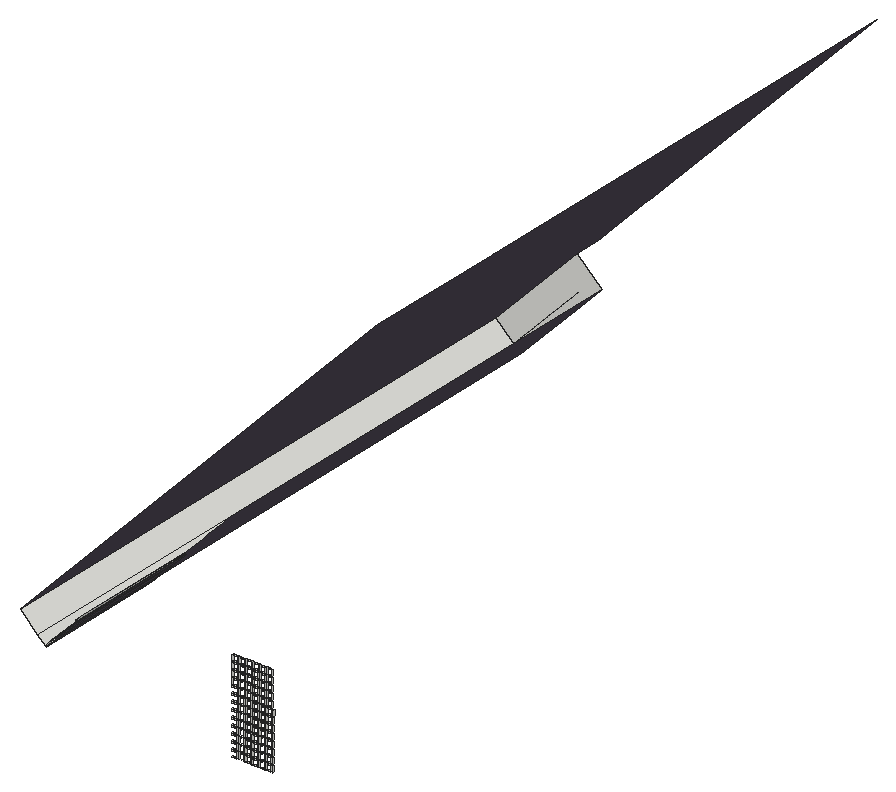
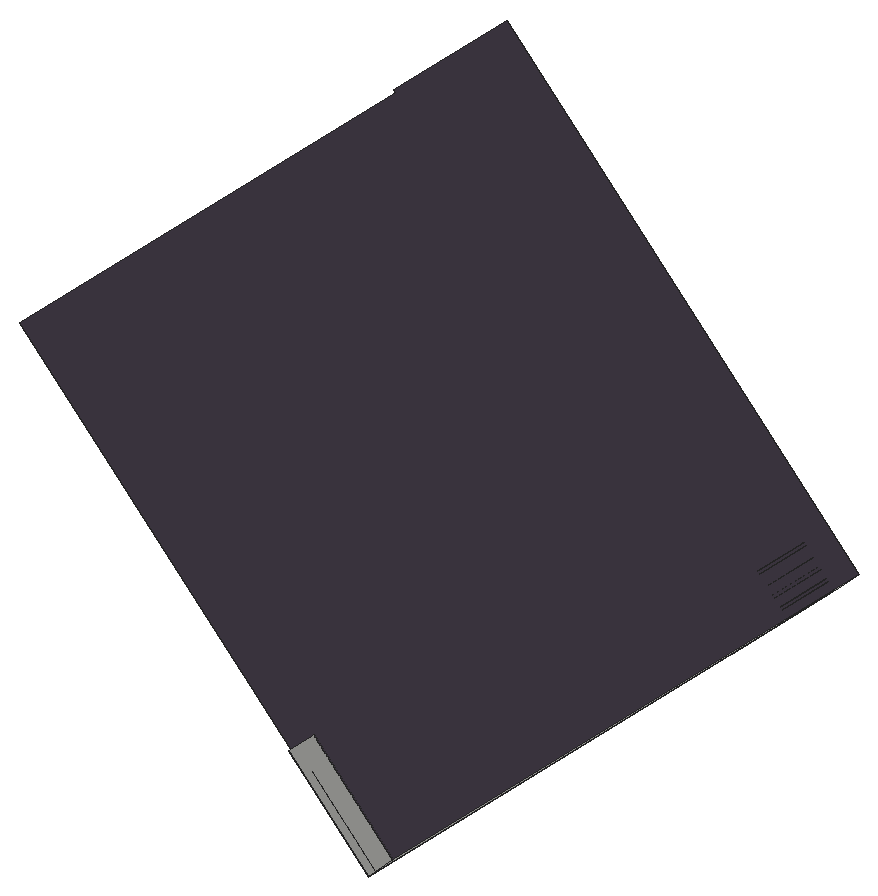
# SketchUp Ruby script. Lengths in inches.
U = 1.inch
M = Sketchup.active_model
def pt(a) = Geom::Point3d.new(a.map { |v| v * U })
def face(e, loops, mat)
  f = e.add_face(loops[0].map { |a| pt(a) })
  loops[1..].each { |l| e.add_face(l.map { |a| pt(a) }).erase! }
  f.material = f.back_material = mat if mat
  f
end
# faces: each face lists its corners as indices into pts; further lists are holes
def faces(e, pts, list, mat = nil) = list.each { |f| face(e, (f[0].is_a?(Array) ? f : [f]).map { |l| l.map { |i| pts[i] } }, mat) }
# xy, xz, yz: faces in a plane at the given z, y or x. An outline is a flat list of corners, or four numbers for a rectangle; further outlines are holes
def ring(l) = l.size == 4 ? [[l[0], l[1]], [l[2], l[1]], [l[2], l[3]], [l[0], l[3]]] : l.each_slice(2).to_a
def flat(e, list, mat, &to3) = list.each { |f| face(e, (f[0].is_a?(Array) ? f : [f]).map { |l| ring(l).map { |u, v| to3.(u, v) } }, mat) }
def xy(e, z, list, mat = nil) = flat(e, list, mat) { |x, y| [x, y, z] }
def xz(e, y, list, mat = nil) = flat(e, list, mat) { |x, z| [x, y, z] }
def yz(e, x, list, mat = nil) = flat(e, list, mat) { |y, z| [x, y, z] }
def lines(e, pts, list) = list.each { |a, b| e.add_line(pt(pts[a]), pt(pts[b])) }
# prism: a flat outline (further loops are holes) pulled along v
def prism(e, loops, v, mat = nil)
  f = face(e, loops, mat); d = Geom::Vector3d.new(v.map { |x| x * U })
  f.pushpull(f.normal.samedirection?(d) ? d.length : -d.length)
end
def box(e, o, s, mat = nil) = prism(e, [[o, [o[0] + s[0], o[1], o[2]], [o[0] + s[0], o[1] + s[1], o[2]], [o[0], o[1] + s[1], o[2]]]], [0, 0, s[2]], mat)
def at(x, y, z, deg = 0) = Geom::Transformation.translation(pt([x, y, z])) * Geom::Transformation.rotation(ORIGIN, Z_AXIS, deg.degrees)
def axes(o, x, y, z) = Geom::Transformation.new([*x, 0, *y, 0, *z, 0, *pt(o).to_a, 1])
def part(name) = M.definitions.add(name)
# library, detail: a bought-in or finely detailed component or shape, given as its bounding box
def library(name, o, s) = part(name).tap { |d| box(d.entities, o, s) }
def detail(e, o, s) = box(e.add_group.entities, o, s)
def put(e, d, t, mat = nil) = e.add_instance(d, t).tap { |i| i.material = mat if mat }
def group(e, t, mat = nil) = e.add_group.tap { |g| g.transformation = t; g.material = mat if mat }.entities
root = M.entities
M.materials.add("[Color M06]").color = [79, 71, 84]
xy(root,265.77,[[989.38,2332.13,991.69,2332.76],[992.29,2332.13,994.6,2332.76],[995.2,2332.13,997.52,2332.76],[998.12,2332.13,1000.43,2332.76],[1001.03,2332.13,1003.34,2332.76],
  [1003.94,2332.13,1006.25,2332.76]])
xy(root,268.09,[[989.38,2332.13,991.69,2332.76],[992.29,2332.13,994.6,2332.76],[995.2,2332.13,997.52,2332.76],[998.12,2332.13,1000.43,2332.76],[1001.03,2332.13,1003.34,2332.76],
  [1003.94,2332.13,1006.25,2332.76]])
xy(root,268.82,[[989.41,2332.13,991.72,2332.76],[992.32,2332.13,994.63,2332.76],[995.23,2332.13,997.55,2332.76],[998.15,2332.13,1000.46,2332.76],[1001.06,2332.13,1003.37,2332.76],
  [1003.97,2332.13,1006.28,2332.76]])
xy(root,271.13,[[989.41,2332.13,991.72,2332.76],[992.32,2332.13,994.63,2332.76],[995.23,2332.13,997.55,2332.76],[998.15,2332.13,1000.46,2332.76],[1001.06,2332.13,1003.37,2332.76],
  [1003.97,2332.13,1006.28,2332.76]])
xy(root,271.86,[[989.4375,2332.13,991.75,2332.76],[992.35,2332.13,994.66,2332.76],[995.26,2332.13,997.57,2332.76],[998.17,2332.13,1000.49,2332.76],[1001.09,2332.13,1003.4,2332.76],
  [1004,2332.13,1006.3125,2332.76]])
xy(root,274.17,[[989.4375,2332.13,991.75,2332.76],[992.35,2332.13,994.66,2332.76],[995.26,2332.13,997.57,2332.76],[998.17,2332.13,1000.49,2332.76],[1001.09,2332.13,1003.4,2332.76],
  [1004,2332.13,1006.3125,2332.76]])
xy(root,274.91,[[989.47,2332.13,991.78,2332.76],[992.38,2332.13,994.69,2332.76],[995.29,2332.13,997.6,2332.76],[998.2,2332.13,1000.52,2332.76],[1001.12,2332.13,1003.43,2332.76],
  [1004.03,2332.13,1006.34,2332.76]])
xy(root,277.22,[[989.47,2332.13,991.78,2332.76],[992.38,2332.13,994.69,2332.76],[995.29,2332.13,997.6,2332.76],[998.2,2332.13,1000.52,2332.76],[1001.12,2332.13,1003.43,2332.76],
  [1004.03,2332.13,1006.34,2332.76]])
xy(root,277.95,[[989.5,2332.13,991.81,2332.76],[992.41,2332.13,994.72,2332.76],[995.32,2332.13,997.63,2332.76],[998.23,2332.13,1000.55,2332.76],[1001.14,2332.13,1003.46,2332.76],
  [1004.06,2332.13,1006.37,2332.76]])
xy(root,280.26,[[989.5,2332.13,991.81,2332.76],[992.41,2332.13,994.72,2332.76],[995.32,2332.13,997.63,2332.76],[998.23,2332.13,1000.55,2332.76],[1001.14,2332.13,1003.46,2332.76],
  [1004.06,2332.13,1006.37,2332.76]])
xy(root,281,[[989.53,2332.13,991.84,2332.76],[992.4375,2332.13,994.75,2332.76],[995.35,2332.13,997.66,2332.76],[998.26,2332.13,1000.57,2332.76],[1001.17,2332.13,1003.49,2332.76],
  [1004.09,2332.13,1006.4,2332.76]])
xy(root,283.31,[[989.53,2332.13,991.84,2332.76],[992.4375,2332.13,994.75,2332.76],[995.35,2332.13,997.66,2332.76],[998.26,2332.13,1000.57,2332.76],[1001.17,2332.13,1003.49,2332.76],
  [1004.09,2332.13,1006.4,2332.76]])
xy(root,284.04,[[989.55,2332.13,991.87,2332.76],[992.47,2332.13,994.78,2332.76],[995.38,2332.13,997.69,2332.76],[998.29,2332.13,1000.6,2332.76],[1001.2,2332.13,1003.52,2332.76],
  [1004.11,2332.13,1006.43,2332.76]])
xy(root,286.35,[[989.55,2332.13,991.87,2332.76],[992.47,2332.13,994.78,2332.76],[995.38,2332.13,997.69,2332.76],[998.29,2332.13,1000.6,2332.76],[1001.2,2332.13,1003.52,2332.76],
  [1004.11,2332.13,1006.43,2332.76]])
xy(root,287.09,[[989.58,2332.13,991.9,2332.76],[992.5,2332.13,994.81,2332.76],[995.41,2332.13,997.72,2332.76],[998.32,2332.13,1000.63,2332.76],[1001.23,2332.13,1003.54,2332.76],
  [1004.14,2332.13,1006.46,2332.76]])
xy(root,289.4,[[989.58,2332.13,991.9,2332.76],[992.5,2332.13,994.81,2332.76],[995.41,2332.13,997.72,2332.76],[998.32,2332.13,1000.63,2332.76],[1001.23,2332.13,1003.54,2332.76],
  [1004.14,2332.13,1006.46,2332.76]])
xy(root,290.13,[[989.61,2332.13,991.92,2332.76],[992.52,2332.13,994.84,2332.76],[995.4375,2332.13,997.75,2332.76],[998.35,2332.13,1000.66,2332.76],[1001.26,2332.13,1003.57,2332.76],
  [1004.17,2332.13,1006.49,2332.76]])
xy(root,292.44,[[989.61,2332.13,991.92,2332.76],[992.52,2332.13,994.84,2332.76],[995.4375,2332.13,997.75,2332.76],[998.35,2332.13,1000.66,2332.76],[1001.26,2332.13,1003.57,2332.76],
  [1004.17,2332.13,1006.49,2332.76]])
xy(root,293.18,[[989.64,2332.13,991.95,2332.76],[992.55,2332.13,994.87,2332.76],[995.47,2332.13,997.78,2332.76],[998.38,2332.13,1000.69,2332.76],[1001.29,2332.13,1003.6,2332.76],
  [1004.2,2332.13,1006.51,2332.76]])
xy(root,295.49,[[989.64,2332.13,991.95,2332.76],[992.55,2332.13,994.87,2332.76],[995.47,2332.13,997.78,2332.76],[998.38,2332.13,1000.69,2332.76],[1001.29,2332.13,1003.6,2332.76],
  [1004.2,2332.13,1006.51,2332.76]])
xy(root,296.22,[[989.67,2332.13,991.98,2332.76],[992.58,2332.13,994.89,2332.76],[995.49,2332.13,997.81,2332.76],[998.41,2332.13,1000.72,2332.76],[1001.32,2332.13,1003.63,2332.76],
  [1004.23,2332.13,1006.54,2332.76]])
xy(root,298.53,[[989.67,2332.13,991.98,2332.76],[992.58,2332.13,994.89,2332.76],[995.49,2332.13,997.81,2332.76],[998.41,2332.13,1000.72,2332.76],[1001.32,2332.13,1003.63,2332.76],
  [1004.23,2332.13,1006.54,2332.76]])
xy(root,299.27,[[989.7,2332.13,992.01,2332.76],[992.61,2332.13,994.92,2332.76],[995.52,2332.13,997.84,2332.76],[998.44,2332.13,1000.75,2332.76],[1001.35,2332.13,1003.66,2332.76],
  [1004.26,2332.13,1006.57,2332.76]])
xy(root,301.58,[[989.7,2332.13,992.01,2332.76],[992.61,2332.13,994.92,2332.76],[995.52,2332.13,997.84,2332.76],[998.44,2332.13,1000.75,2332.76],[1001.35,2332.13,1003.66,2332.76],
  [1004.26,2332.13,1006.57,2332.76]])
xy(root,302.31,[[989.73,2332.13,992.04,2332.76],[992.64,2332.13,994.95,2332.76],[995.55,2332.13,997.86,2332.76],[998.46,2332.13,1000.78,2332.76],[1001.375,2332.13,1003.6875,2332.76],
  [1004.29,2332.13,1006.6,2332.76]])
xy(root,304.62,[[989.73,2332.13,992.04,2332.76],[992.64,2332.13,994.95,2332.76],[995.55,2332.13,997.86,2332.76],[998.46,2332.13,1000.78,2332.76],[1001.375,2332.13,1003.6875,2332.76],
  [1004.29,2332.13,1006.6,2332.76]])
xz(root,2373.56,[[921.31,289.13,920.85,289.56,923.27,292.13,923.73,291.7],[924.61,292.64,924.15,293.0625,926.57,295.64,927.03,295.21],[927.91,296.14,927.45,296.57,929.87,299.14,930.33,298.71],[931.2,299.64,930.75,300.07,933.17,302.64,933.625,302.22],[934.5,303.15,934.05,303.58,936.47,306.15,936.92,305.72],
  [934.05,303.58,933.82,303.79,936.24,306.36,936.47,306.15]])
xz(root,2571.2,[[920.85,289.56,917.71,292.52,910.18,299.61,944.56,336.13,955.23,326.08,948.3125,318.73]])
yz(root,989.64,[[2332.13,293.18,2332.76,295.49]])
yz(root,989.67,[[2332.13,296.22,2332.76,298.53]])
yz(root,989.7,[[2332.13,299.27,2332.76,301.58]])
yz(root,989.73,[[2332.13,302.31,2332.76,304.62]])
yz(root,991.69,[[2332.13,265.77,2332.76,268.09]])
yz(root,991.72,[[2332.13,268.82,2332.76,271.13]])
yz(root,991.75,[[2332.13,271.86,2332.76,274.17]])
yz(root,991.78,[[2332.13,274.91,2332.76,277.22]])
yz(root,991.81,[[2332.13,277.95,2332.76,280.26]])
yz(root,991.84,[[2332.13,281,2332.76,283.31]])
yz(root,991.87,[[2332.13,284.04,2332.76,286.35]])
yz(root,991.9,[[2332.13,287.09,2332.76,289.4]])
yz(root,991.92,[[2332.13,290.13,2332.76,292.44]])
yz(root,991.95,[[2332.13,293.18,2332.76,295.49]])
yz(root,991.98,[[2332.13,296.22,2332.76,298.53]])
yz(root,992.01,[[2332.13,299.27,2332.76,301.58]])
yz(root,992.04,[[2332.13,302.31,2332.76,304.62]])
yz(root,992.29,[[2332.13,265.77,2332.76,268.09]])
yz(root,992.32,[[2332.13,268.82,2332.76,271.13]])
yz(root,992.35,[[2332.13,271.86,2332.76,274.17]])
yz(root,992.38,[[2332.13,274.91,2332.76,277.22]])
yz(root,992.41,[[2332.13,277.95,2332.76,280.26]])
yz(root,992.4375,[[2332.13,281,2332.76,283.31]])
yz(root,992.47,[[2332.13,284.04,2332.76,286.35]])
yz(root,992.5,[[2332.13,287.09,2332.76,289.4]])
yz(root,992.52,[[2332.13,290.13,2332.76,292.44]])
yz(root,992.55,[[2332.13,293.18,2332.76,295.49]])
yz(root,992.58,[[2332.13,296.22,2332.76,298.53]])
yz(root,992.61,[[2332.13,299.27,2332.76,301.58]])
yz(root,992.64,[[2332.13,302.31,2332.76,304.62]])
yz(root,994.6,[[2332.13,265.77,2332.76,268.09]])
yz(root,994.63,[[2332.13,268.82,2332.76,271.13]])
yz(root,994.66,[[2332.13,271.86,2332.76,274.17]])
yz(root,994.69,[[2332.13,274.91,2332.76,277.22]])
yz(root,994.72,[[2332.13,277.95,2332.76,280.26]])
yz(root,994.75,[[2332.13,281,2332.76,283.31]])
yz(root,994.78,[[2332.13,284.04,2332.76,286.35]])
yz(root,994.81,[[2332.13,287.09,2332.76,289.4]])
yz(root,994.84,[[2332.13,290.13,2332.76,292.44]])
yz(root,994.87,[[2332.13,293.18,2332.76,295.49]])
yz(root,994.89,[[2332.13,296.22,2332.76,298.53]])
yz(root,994.92,[[2332.13,299.27,2332.76,301.58]])
yz(root,994.95,[[2332.13,302.31,2332.76,304.62]])
yz(root,995.2,[[2332.13,265.77,2332.76,268.09]])
yz(root,995.23,[[2332.13,268.82,2332.76,271.13]])
yz(root,995.26,[[2332.13,271.86,2332.76,274.17]])
yz(root,995.29,[[2332.13,274.91,2332.76,277.22]])
yz(root,995.32,[[2332.13,277.95,2332.76,280.26]])
yz(root,995.35,[[2332.13,281,2332.76,283.31]])
yz(root,995.38,[[2332.13,284.04,2332.76,286.35]])
yz(root,995.41,[[2332.13,287.09,2332.76,289.4]])
yz(root,995.4375,[[2332.13,290.13,2332.76,292.44]])
yz(root,995.47,[[2332.13,293.18,2332.76,295.49]])
yz(root,995.49,[[2332.13,296.22,2332.76,298.53]])
yz(root,995.52,[[2332.13,299.27,2332.76,301.58]])
yz(root,995.55,[[2332.13,302.31,2332.76,304.62]])
yz(root,997.52,[[2332.13,265.77,2332.76,268.09]])
yz(root,997.55,[[2332.13,268.82,2332.76,271.13]])
yz(root,997.57,[[2332.13,271.86,2332.76,274.17]])
yz(root,997.6,[[2332.13,274.91,2332.76,277.22]])
yz(root,997.63,[[2332.13,277.95,2332.76,280.26]])
yz(root,997.66,[[2332.13,281,2332.76,283.31]])
yz(root,997.69,[[2332.13,284.04,2332.76,286.35]])
yz(root,997.72,[[2332.13,287.09,2332.76,289.4]])
yz(root,997.75,[[2332.13,290.13,2332.76,292.44]])
yz(root,997.78,[[2332.13,293.18,2332.76,295.49]])
yz(root,997.81,[[2332.13,296.22,2332.76,298.53]])
yz(root,997.84,[[2332.13,299.27,2332.76,301.58]])
yz(root,997.86,[[2332.13,302.31,2332.76,304.62]])
yz(root,998.12,[[2332.13,265.77,2332.76,268.09]])
yz(root,998.15,[[2332.13,268.82,2332.76,271.13]])
yz(root,998.17,[[2332.13,271.86,2332.76,274.17]])
yz(root,998.2,[[2332.13,274.91,2332.76,277.22]])
yz(root,998.23,[[2332.13,277.95,2332.76,280.26]])
yz(root,998.26,[[2332.13,281,2332.76,283.31]])
yz(root,998.29,[[2332.13,284.04,2332.76,286.35]])
yz(root,998.32,[[2332.13,287.09,2332.76,289.4]])
yz(root,998.35,[[2332.13,290.13,2332.76,292.44]])
yz(root,998.38,[[2332.13,293.18,2332.76,295.49]])
yz(root,998.41,[[2332.13,296.22,2332.76,298.53]])
yz(root,998.44,[[2332.13,299.27,2332.76,301.58]])
yz(root,998.46,[[2332.13,302.31,2332.76,304.62]])
yz(root,1000.43,[[2332.13,265.77,2332.76,268.09]])
yz(root,1000.46,[[2332.13,268.82,2332.76,271.13]])
yz(root,1000.49,[[2332.13,271.86,2332.76,274.17]])
yz(root,1000.52,[[2332.13,274.91,2332.76,277.22]])
yz(root,1000.55,[[2332.13,277.95,2332.76,280.26]])
yz(root,1000.57,[[2332.13,281,2332.76,283.31]])
yz(root,1000.6,[[2332.13,284.04,2332.76,286.35]])
yz(root,1000.63,[[2332.13,287.09,2332.76,289.4]])
yz(root,1000.66,[[2332.13,290.13,2332.76,292.44]])
yz(root,1000.69,[[2332.13,293.18,2332.76,295.49]])
yz(root,1000.72,[[2332.13,296.22,2332.76,298.53]])
yz(root,1000.75,[[2332.13,299.27,2332.76,301.58]])
yz(root,1000.78,[[2332.13,302.31,2332.76,304.62]])
yz(root,1001.03,[[2332.13,265.77,2332.76,268.09]])
yz(root,1001.06,[[2332.13,268.82,2332.76,271.13]])
yz(root,1001.09,[[2332.13,271.86,2332.76,274.17]])
yz(root,1001.12,[[2332.13,274.91,2332.76,277.22]])
yz(root,1001.14,[[2332.13,277.95,2332.76,280.26]])
yz(root,1001.17,[[2332.13,281,2332.76,283.31]])
yz(root,1001.2,[[2332.13,284.04,2332.76,286.35]])
yz(root,1001.23,[[2332.13,287.09,2332.76,289.4]])
yz(root,1001.26,[[2332.13,290.13,2332.76,292.44]])
yz(root,1001.29,[[2332.13,293.18,2332.76,295.49]])
yz(root,1001.32,[[2332.13,296.22,2332.76,298.53]])
yz(root,1001.35,[[2332.13,299.27,2332.76,301.58]])
yz(root,1001.375,[[2332.13,302.31,2332.76,304.62]])
yz(root,1003.34,[[2332.13,265.77,2332.76,268.09]])
yz(root,1003.37,[[2332.13,268.82,2332.76,271.13]])
yz(root,1003.4,[[2332.13,271.86,2332.76,274.17]])
yz(root,1003.43,[[2332.13,274.91,2332.76,277.22]])
yz(root,1003.46,[[2332.13,277.95,2332.76,280.26]])
yz(root,1003.49,[[2332.13,281,2332.76,283.31]])
yz(root,1003.52,[[2332.13,284.04,2332.76,286.35]])
yz(root,1003.54,[[2332.13,287.09,2332.76,289.4]])
yz(root,1003.57,[[2332.13,290.13,2332.76,292.44]])
yz(root,1003.6,[[2332.13,293.18,2332.76,295.49]])
yz(root,1003.63,[[2332.13,296.22,2332.76,298.53]])
yz(root,1003.66,[[2332.13,299.27,2332.76,301.58]])
yz(root,1003.6875,[[2332.13,302.31,2332.76,304.62]])
yz(root,1003.94,[[2332.13,265.77,2332.76,268.09]])
yz(root,1003.97,[[2332.13,268.82,2332.76,271.13]])
yz(root,1004,[[2332.13,271.86,2332.76,274.17]])
yz(root,1004.03,[[2332.13,274.91,2332.76,277.22]])
yz(root,1004.06,[[2332.13,277.95,2332.76,280.26]])
yz(root,1004.09,[[2332.13,281,2332.76,283.31]])
yz(root,1004.11,[[2332.13,284.04,2332.76,286.35]])
yz(root,1004.14,[[2332.13,287.09,2332.76,289.4]])
yz(root,1004.17,[[2332.13,290.13,2332.76,292.44]])
yz(root,1004.2,[[2332.13,293.18,2332.76,295.49]])
yz(root,1004.23,[[2332.13,296.22,2332.76,298.53]])
yz(root,1004.26,[[2332.13,299.27,2332.76,301.58]])
yz(root,1004.29,[[2332.13,302.31,2332.76,304.62]])
yz(root,1006.25,[[2332.13,265.77,2332.76,268.09]])
yz(root,1006.28,[[2332.13,268.82,2332.76,271.13]])
yz(root,1006.3125,[[2332.13,271.86,2332.76,274.17]])
yz(root,1006.34,[[2332.13,274.91,2332.76,277.22]])
yz(root,1006.37,[[2332.13,277.95,2332.76,280.26]])
yz(root,1006.4,[[2332.13,281,2332.76,283.31]])
yz(root,1006.43,[[2332.13,284.04,2332.76,286.35]])
yz(root,1006.46,[[2332.13,287.09,2332.76,289.4]])
yz(root,1006.49,[[2332.13,290.13,2332.76,292.44]])
yz(root,1006.51,[[2332.13,293.18,2332.76,295.49]])
yz(root,1006.54,[[2332.13,296.22,2332.76,298.53]])
yz(root,1006.57,[[2332.13,299.27,2332.76,301.58]])
yz(root,1006.6,[[2332.13,302.31,2332.76,304.62]])
yz(root,1006.85,[[2332.13,265.77,2332.76,268.09]])
yz(root,1006.88,[[2332.13,268.82,2332.76,271.13]])
yz(root,1006.91,[[2332.13,271.86,2332.76,274.17]])
yz(root,1006.94,[[2332.13,274.91,2332.76,277.22]])
yz(root,1006.97,[[2332.13,277.95,2332.76,280.26]])
yz(root,1007,[[2332.13,281,2332.76,283.31]])
yz(root,1007.03,[[2332.13,284.04,2332.76,286.35]])
yz(root,1007.06,[[2332.13,287.09,2332.76,289.4]])
p = [[920.85,2319.18,289.56],[920.85,2373.56,289.56],[921.31,2373.56,289.13],[921.31,2319.18,289.13],[923.73,2373.56,291.7],[923.73,2319.18,291.7],
  [917.71,2319.18,292.52],[917.71,2380.48,292.52],[917.71,2571.2,292.52],[920.85,2571.2,289.56],[923.27,2373.56,292.13],[923.27,2319.18,292.13],
  [955.23,2571.2,326.08],[955.23,2380.48,326.08],[955.23,2373.56,326.08],[953.84,2373.56,324.6],[952.96,2373.56,323.67],[950.54,2373.56,321.1],
  [949.66,2373.56,320.17],[948.3125,2373.56,318.73],[947.24,2373.56,317.59],[946.36,2373.56,316.66],[943.94,2373.56,314.09],[943.07,2373.56,313.16],
  [940.64,2373.56,310.59],[939.77,2373.56,309.65],[937.35,2373.56,307.08],[936.47,2373.56,306.15],[934.05,2373.56,303.58],[933.17,2373.56,302.64],
  [930.75,2373.56,300.07],[929.87,2373.56,299.14],[927.45,2373.56,296.57],[926.57,2373.56,295.64],[924.15,2373.56,293.0625],[948.3125,2571.2,318.73],
  [924.15,2319.18,293.0625],[910.18,2319.18,299.61],[910.18,2571.2,299.61],[924.61,2373.56,292.64],[924.61,2319.18,292.64],[927.03,2373.56,295.21],
  [927.03,2319.18,295.21],[926.57,2319.18,295.64],[927.45,2319.18,296.57],[927.91,2373.56,296.14],[927.91,2319.18,296.14],[930.33,2373.56,298.71],
  [930.33,2319.18,298.71],[929.87,2319.18,299.14],[930.75,2319.18,300.07],[1062.38,2319.18,461.31],[1062.38,2380.48,461.31],[1061.61,2380.48,460.49],
  [1061.61,2583.74,460.49],[965.61,2583.74,358.5],[964.88,2583.74,357.73],[948.3125,2583.74,340.125],[944.56,2583.74,336.13],[944.56,2571.2,336.13],
  [931.2,2373.56,299.64],[931.2,2319.18,299.64],[933.625,2373.56,302.22],[933.625,2319.18,302.22],[933.17,2319.18,302.64],[934.05,2319.18,303.58],
  [934.5,2373.56,303.15],[934.5,2319.18,303.15],[936.92,2373.56,305.72],[936.92,2319.18,305.72],[933.82,2319.18,303.79],[933.82,2373.56,303.79],
  [936.47,2319.18,306.15],[936.24,2373.56,306.36],[936.24,2319.18,306.36],[945.17,2571.2,321.6875]]
faces(root,p,[[0,1,2,3],[0,6,7,8,9,1],[10,1,0,11],[10,11,5,4],[6,37,38,8,7],[36,34,39,40],[33,34,36,43],[33,43,42,41],
  [44,32,45,46],[31,32,44,49],[31,49,48,47],[50,30,60,61],[29,30,50,64],[29,64,63,62],[28,65,70,71],[27,28,65,72],
  [73,71,70,74]])
faces(root,p,[[2,4,5,3],[12,13,14,15,16,17,18,19,20,21,22,23,24,25,26,27,28,29,30,31,32,33,34,10,1,9,35],[10,34,36,11],[39,41,42,40],[33,32,44,43],[45,47,48,46],[31,30,50,49],[38,37,51,52,53,54,55,56,57,58,59],
  [60,62,63,61],[29,28,65,64],[65,28,66,67],[66,68,69,67]],"[Color M06]")
lines(root,p,[[75,8]])
